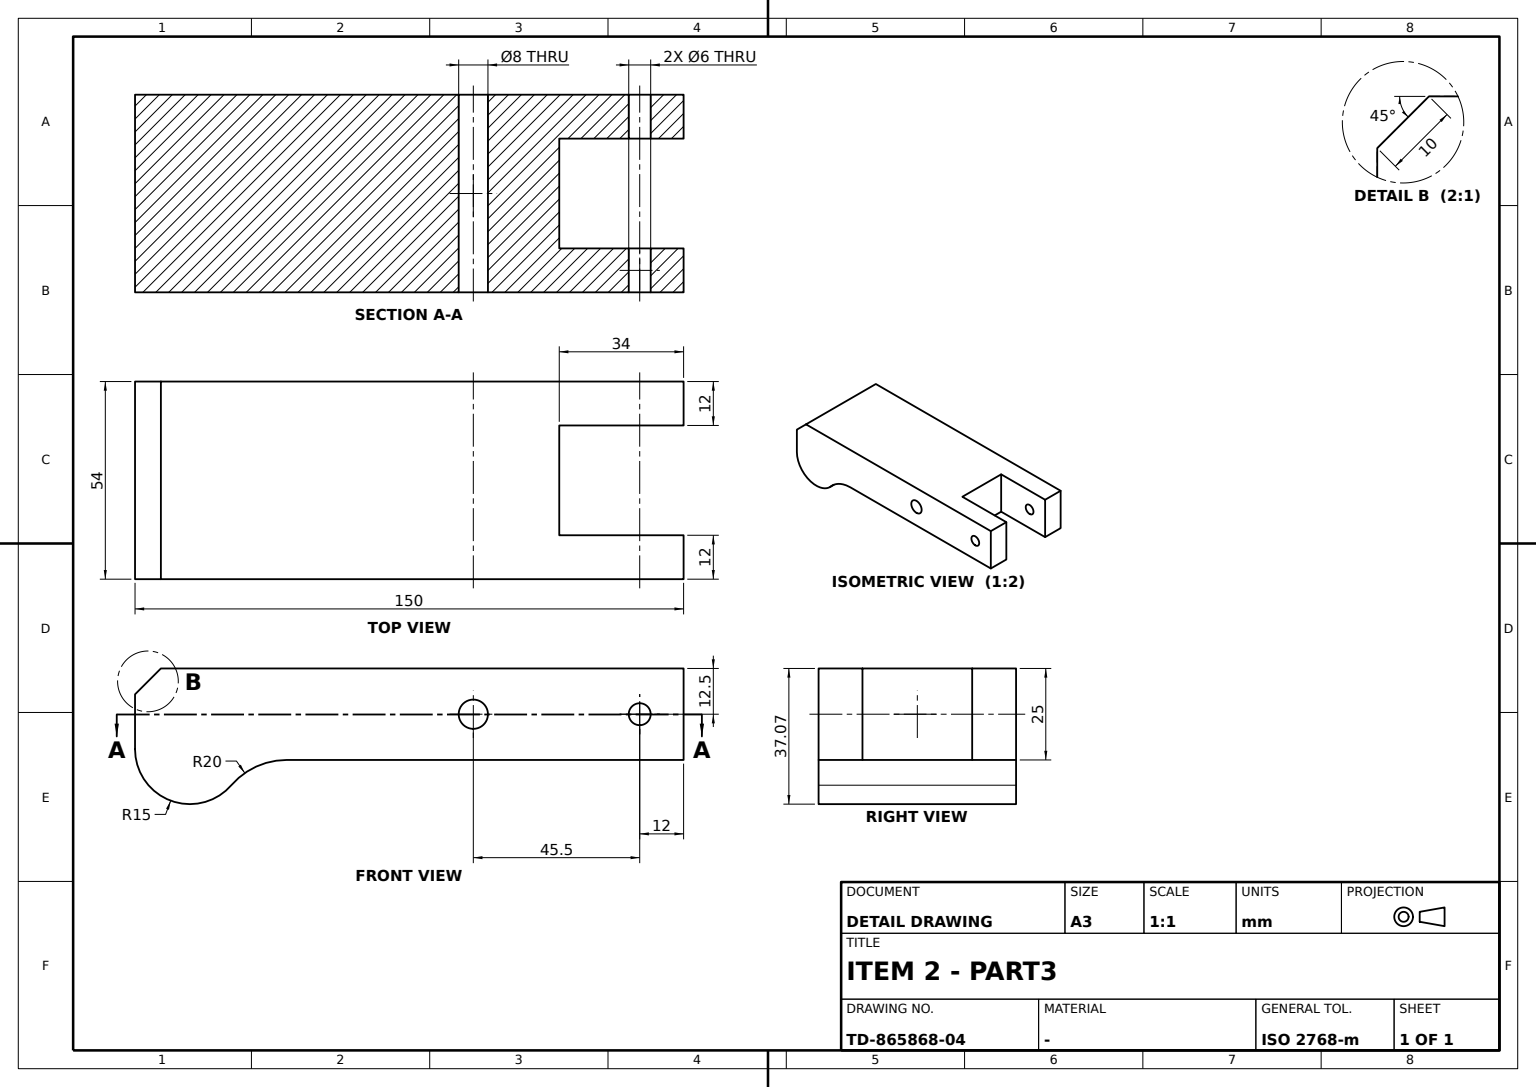
ISO-10303-21;
HEADER;
FILE_DESCRIPTION((''),'2;1');
FILE_NAME('','',(''),(''),'','','');
FILE_SCHEMA(('AUTOMOTIVE_DESIGN'));
ENDSEC;
DATA;
#1=APPLICATION_CONTEXT('');
#2=PRODUCT_CONTEXT('',#1,'mechanical');
#3=PRODUCT('','','',(#2));
#4=PRODUCT_DEFINITION_FORMATION('','',#3);
#5=PRODUCT_DEFINITION_CONTEXT('',#1,'design');
#6=PRODUCT_DEFINITION('','',#4,#5);
#7=PRODUCT_DEFINITION_SHAPE('','',#6);
#8=(LENGTH_UNIT()NAMED_UNIT(*)SI_UNIT(.MILLI.,.METRE.));
#9=(NAMED_UNIT(*)PLANE_ANGLE_UNIT()SI_UNIT($,.RADIAN.));
#10=(NAMED_UNIT(*)SI_UNIT($,.STERADIAN.)SOLID_ANGLE_UNIT());
#11=UNCERTAINTY_MEASURE_WITH_UNIT(LENGTH_MEASURE(0.005),#8,'distance_accuracy_value','');
#12=(GEOMETRIC_REPRESENTATION_CONTEXT(3)GLOBAL_UNCERTAINTY_ASSIGNED_CONTEXT((#11))GLOBAL_UNIT_ASSIGNED_CONTEXT((#8,#9,#10))REPRESENTATION_CONTEXT('',''));
#13=CARTESIAN_POINT('',(27.,77.5,5.571068));
#14=VERTEX_POINT('',#13);
#15=CARTESIAN_POINT('',(27.,77.5,9.571068));
#16=DIRECTION('',(1.,0.,0.));
#17=DIRECTION('',(0.,0.,-1.));
#18=AXIS2_PLACEMENT_3D('',#15,#16,#17);
#19=CIRCLE('',#18,4.);
#20=EDGE_CURVE('',#14,#14,#19,.T.);
#21=ORIENTED_EDGE('',*,*,#20,.T.);
#22=EDGE_LOOP('',(#21));
#23=FACE_BOUND('',#22,.T.);
#24=CARTESIAN_POINT('',(-27.,77.5,5.571068));
#25=VERTEX_POINT('',#24);
#26=CARTESIAN_POINT('',(-27.,77.5,9.571068));
#27=AXIS2_PLACEMENT_3D('',#26,#16,#17);
#28=CIRCLE('',#27,4.);
#29=EDGE_CURVE('',#25,#25,#28,.T.);
#30=ORIENTED_EDGE('',*,*,#29,.F.);
#31=EDGE_LOOP('',(#30));
#32=FACE_BOUND('',#31,.T.);
#33=CARTESIAN_POINT('',(-0.66,77.5,9.571068));
#34=DIRECTION('',(0.,1.,0.));
#35=AXIS2_PLACEMENT_3D('',#33,#16,#34);
#36=CYLINDRICAL_SURFACE('',#35,4.);
#37=ADVANCED_FACE('',(#23,#32),#36,.F.);
#38=CARTESIAN_POINT('',(15.,101.,22.071068));
#39=VERTEX_POINT('',#38);
#40=CARTESIAN_POINT('',(15.,101.,-2.928932));
#41=VERTEX_POINT('',#40);
#42=VECTOR('',#17,1000.);
#43=LINE('',#38,#42);
#44=EDGE_CURVE('',#39,#41,#43,.T.);
#45=ORIENTED_EDGE('',*,*,#44,.T.);
#46=CARTESIAN_POINT('',(-15.,101.,-2.928932));
#47=VERTEX_POINT('',#46);
#48=DIRECTION('',(-1.,0.,0.));
#49=VECTOR('',#48,1000.);
#50=LINE('',#40,#49);
#51=EDGE_CURVE('',#41,#47,#50,.T.);
#52=ORIENTED_EDGE('',*,*,#51,.T.);
#53=CARTESIAN_POINT('',(-15.,101.,22.071068));
#54=VERTEX_POINT('',#53);
#55=LINE('',#53,#42);
#56=EDGE_CURVE('',#54,#47,#55,.T.);
#57=ORIENTED_EDGE('',*,*,#56,.F.);
#58=CARTESIAN_POINT('',(0.,101.,22.071068));
#59=LINE('',#58,#49);
#60=EDGE_CURVE('',#39,#54,#59,.T.);
#61=ORIENTED_EDGE('',*,*,#60,.F.);
#62=EDGE_LOOP('',(#45,#52,#57,#61));
#63=FACE_BOUND('',#62,.T.);
#64=DIRECTION('',(0.,-1.,0.));
#65=AXIS2_PLACEMENT_3D('',#38,#64,#48);
#66=PLANE('',#65);
#67=ADVANCED_FACE('',(#63),#66,.F.);
#68=CARTESIAN_POINT('',(15.,135.,-2.928932));
#69=VERTEX_POINT('',#68);
#70=CARTESIAN_POINT('',(27.,135.,-2.928932));
#71=VERTEX_POINT('',#70);
#72=CARTESIAN_POINT('',(0.,135.,-2.928932));
#73=VECTOR('',#16,1000.);
#74=LINE('',#72,#73);
#75=EDGE_CURVE('',#69,#71,#74,.T.);
#76=ORIENTED_EDGE('',*,*,#75,.T.);
#77=CARTESIAN_POINT('',(27.,26.443602,-2.928932));
#78=VERTEX_POINT('',#77);
#79=CARTESIAN_POINT('',(27.,0.,-2.928932));
#80=VECTOR('',#64,1000.);
#81=LINE('',#79,#80);
#82=EDGE_CURVE('',#71,#78,#81,.T.);
#83=ORIENTED_EDGE('',*,*,#82,.T.);
#84=CARTESIAN_POINT('',(-27.,26.443602,-2.928932));
#85=VERTEX_POINT('',#84);
#86=CARTESIAN_POINT('',(0.,26.443602,-2.928932));
#87=LINE('',#86,#73);
#88=EDGE_CURVE('',#85,#78,#87,.T.);
#89=ORIENTED_EDGE('',*,*,#88,.F.);
#90=CARTESIAN_POINT('',(-27.,135.,-2.928932));
#91=VERTEX_POINT('',#90);
#92=CARTESIAN_POINT('',(-27.,0.,-2.928932));
#93=LINE('',#92,#80);
#94=EDGE_CURVE('',#91,#85,#93,.T.);
#95=ORIENTED_EDGE('',*,*,#94,.F.);
#96=CARTESIAN_POINT('',(-15.,135.,-2.928932));
#97=VERTEX_POINT('',#96);
#98=EDGE_CURVE('',#91,#97,#74,.T.);
#99=ORIENTED_EDGE('',*,*,#98,.T.);
#100=LINE('',#96,#80);
#101=EDGE_CURVE('',#97,#47,#100,.T.);
#102=ORIENTED_EDGE('',*,*,#101,.T.);
#103=ORIENTED_EDGE('',*,*,#51,.F.);
#104=LINE('',#68,#80);
#105=EDGE_CURVE('',#69,#41,#104,.T.);
#106=ORIENTED_EDGE('',*,*,#105,.F.);
#107=EDGE_LOOP('',(#76,#83,#89,#95,#99,#102,#103,#106));
#108=FACE_BOUND('',#107,.T.);
#109=DIRECTION('',(0.,0.,1.));
#110=AXIS2_PLACEMENT_3D('',#72,#109,#64);
#111=PLANE('',#110);
#112=ADVANCED_FACE('',(#108),#111,.F.);
#113=CARTESIAN_POINT('',(27.,-15.,15.));
#114=VERTEX_POINT('',#113);
#115=CARTESIAN_POINT('',(27.,-7.928932,22.071068));
#116=VERTEX_POINT('',#115);
#117=DIRECTION('',(0.,0.707106781,0.707106781));
#118=VECTOR('',#117,1000.);
#119=LINE('',#113,#118);
#120=EDGE_CURVE('',#114,#116,#119,.T.);
#121=ORIENTED_EDGE('',*,*,#120,.T.);
#122=CARTESIAN_POINT('',(-27.,-7.928932,22.071068));
#123=VERTEX_POINT('',#122);
#124=CARTESIAN_POINT('',(0.,-7.928932,22.071068));
#125=LINE('',#124,#73);
#126=EDGE_CURVE('',#123,#116,#125,.T.);
#127=ORIENTED_EDGE('',*,*,#126,.F.);
#128=CARTESIAN_POINT('',(-27.,-15.,15.));
#129=VERTEX_POINT('',#128);
#130=LINE('',#128,#118);
#131=EDGE_CURVE('',#129,#123,#130,.T.);
#132=ORIENTED_EDGE('',*,*,#131,.F.);
#133=CARTESIAN_POINT('',(0.,-15.,15.));
#134=LINE('',#133,#73);
#135=EDGE_CURVE('',#129,#114,#134,.T.);
#136=ORIENTED_EDGE('',*,*,#135,.T.);
#137=EDGE_LOOP('',(#121,#127,#132,#136));
#138=FACE_BOUND('',#137,.T.);
#139=DIRECTION('',(0.,0.707106781,-0.707106781));
#140=AXIS2_PLACEMENT_3D('',#133,#139,#117);
#141=PLANE('',#140);
#142=ADVANCED_FACE('',(#138),#141,.F.);
#143=CARTESIAN_POINT('',(-27.,123.,6.571068));
#144=VERTEX_POINT('',#143);
#145=CARTESIAN_POINT('',(-27.,123.,9.571068));
#146=AXIS2_PLACEMENT_3D('',#145,#16,#17);
#147=CIRCLE('',#146,3.);
#148=EDGE_CURVE('',#144,#144,#147,.T.);
#149=ORIENTED_EDGE('',*,*,#148,.T.);
#150=EDGE_LOOP('',(#149));
#151=FACE_BOUND('',#150,.T.);
#152=CARTESIAN_POINT('',(-27.,135.,22.071068));
#153=VERTEX_POINT('',#152);
#154=CARTESIAN_POINT('',(-27.,0.,22.071068));
#155=VECTOR('',#34,1000.);
#156=LINE('',#154,#155);
#157=EDGE_CURVE('',#123,#153,#156,.T.);
#158=ORIENTED_EDGE('',*,*,#157,.T.);
#159=CARTESIAN_POINT('',(-27.,135.,0.));
#160=LINE('',#159,#42);
#161=EDGE_CURVE('',#153,#91,#160,.T.);
#162=ORIENTED_EDGE('',*,*,#161,.T.);
#163=ORIENTED_EDGE('',*,*,#94,.T.);
#164=CARTESIAN_POINT('',(-27.,11.332972,-9.826685));
#165=VERTEX_POINT('',#164);
#166=CARTESIAN_POINT('',(-27.,26.443602,-22.928932));
#167=AXIS2_PLACEMENT_3D('',#166,#16,#17);
#168=CIRCLE('',#167,20.);
#169=EDGE_CURVE('',#85,#165,#168,.T.);
#170=ORIENTED_EDGE('',*,*,#169,.T.);
#171=CARTESIAN_POINT('',(-27.,-15.,0.));
#172=VERTEX_POINT('',#171);
#173=CARTESIAN_POINT('',(-27.,0.,0.));
#174=AXIS2_PLACEMENT_3D('',#173,#16,#17);
#175=CIRCLE('',#174,15.);
#176=EDGE_CURVE('',#172,#165,#175,.T.);
#177=ORIENTED_EDGE('',*,*,#176,.F.);
#178=VECTOR('',#109,1000.);
#179=LINE('',#171,#178);
#180=EDGE_CURVE('',#172,#129,#179,.T.);
#181=ORIENTED_EDGE('',*,*,#180,.T.);
#182=ORIENTED_EDGE('',*,*,#131,.T.);
#183=EDGE_LOOP('',(#158,#162,#163,#170,#177,#181,#182));
#184=FACE_BOUND('',#183,.T.);
#185=ORIENTED_EDGE('',*,*,#29,.T.);
#186=EDGE_LOOP('',(#185));
#187=FACE_BOUND('',#186,.T.);
#188=AXIS2_PLACEMENT_3D('',#173,#16,#34);
#189=PLANE('',#188);
#190=ADVANCED_FACE('',(#151,#184,#187),#189,.F.);
#191=ORIENTED_EDGE('',*,*,#56,.T.);
#192=ORIENTED_EDGE('',*,*,#101,.F.);
#193=CARTESIAN_POINT('',(-15.,135.,22.071068));
#194=VERTEX_POINT('',#193);
#195=LINE('',#193,#42);
#196=EDGE_CURVE('',#194,#97,#195,.T.);
#197=ORIENTED_EDGE('',*,*,#196,.F.);
#198=CARTESIAN_POINT('',(-15.,-7.928932,22.071068));
#199=LINE('',#198,#155);
#200=EDGE_CURVE('',#54,#194,#199,.T.);
#201=ORIENTED_EDGE('',*,*,#200,.F.);
#202=EDGE_LOOP('',(#191,#192,#197,#201));
#203=FACE_BOUND('',#202,.T.);
#204=CARTESIAN_POINT('',(-15.,123.,12.571068));
#205=VERTEX_POINT('',#204);
#206=CARTESIAN_POINT('',(-15.,123.,9.571068));
#207=AXIS2_PLACEMENT_3D('',#206,#48,#109);
#208=CIRCLE('',#207,3.);
#209=EDGE_CURVE('',#205,#205,#208,.T.);
#210=ORIENTED_EDGE('',*,*,#209,.T.);
#211=EDGE_LOOP('',(#210));
#212=FACE_BOUND('',#211,.T.);
#213=AXIS2_PLACEMENT_3D('',#53,#48,#34);
#214=PLANE('',#213);
#215=ADVANCED_FACE('',(#203,#212),#214,.F.);
#216=ORIENTED_EDGE('',*,*,#209,.F.);
#217=EDGE_LOOP('',(#216));
#218=FACE_BOUND('',#217,.T.);
#219=ORIENTED_EDGE('',*,*,#148,.F.);
#220=EDGE_LOOP('',(#219));
#221=FACE_BOUND('',#220,.T.);
#222=CARTESIAN_POINT('',(-0.66,123.,9.571068));
#223=AXIS2_PLACEMENT_3D('',#222,#16,#34);
#224=CYLINDRICAL_SURFACE('',#223,3.);
#225=ADVANCED_FACE('',(#218,#221),#224,.F.);
#226=CARTESIAN_POINT('',(15.,135.,22.071068));
#227=VERTEX_POINT('',#226);
#228=CARTESIAN_POINT('',(27.,135.,22.071068));
#229=VERTEX_POINT('',#228);
#230=CARTESIAN_POINT('',(0.,135.,22.071068));
#231=LINE('',#230,#73);
#232=EDGE_CURVE('',#227,#229,#231,.T.);
#233=ORIENTED_EDGE('',*,*,#232,.T.);
#234=CARTESIAN_POINT('',(27.,135.,0.));
#235=LINE('',#234,#42);
#236=EDGE_CURVE('',#229,#71,#235,.T.);
#237=ORIENTED_EDGE('',*,*,#236,.T.);
#238=ORIENTED_EDGE('',*,*,#75,.F.);
#239=LINE('',#226,#42);
#240=EDGE_CURVE('',#227,#69,#239,.T.);
#241=ORIENTED_EDGE('',*,*,#240,.F.);
#242=EDGE_LOOP('',(#233,#237,#238,#241));
#243=FACE_BOUND('',#242,.T.);
#244=AXIS2_PLACEMENT_3D('',#230,#64,#17);
#245=PLANE('',#244);
#246=ADVANCED_FACE('',(#243),#245,.F.);
#247=EDGE_CURVE('',#153,#194,#231,.T.);
#248=ORIENTED_EDGE('',*,*,#247,.F.);
#249=ORIENTED_EDGE('',*,*,#157,.F.);
#250=ORIENTED_EDGE('',*,*,#126,.T.);
#251=CARTESIAN_POINT('',(27.,0.,22.071068));
#252=LINE('',#251,#155);
#253=EDGE_CURVE('',#116,#229,#252,.T.);
#254=ORIENTED_EDGE('',*,*,#253,.T.);
#255=ORIENTED_EDGE('',*,*,#232,.F.);
#256=CARTESIAN_POINT('',(15.,-7.928932,22.071068));
#257=LINE('',#256,#80);
#258=EDGE_CURVE('',#227,#39,#257,.T.);
#259=ORIENTED_EDGE('',*,*,#258,.T.);
#260=ORIENTED_EDGE('',*,*,#60,.T.);
#261=ORIENTED_EDGE('',*,*,#200,.T.);
#262=EDGE_LOOP('',(#248,#249,#250,#254,#255,#259,#260,#261));
#263=FACE_BOUND('',#262,.T.);
#264=AXIS2_PLACEMENT_3D('',#124,#17,#34);
#265=PLANE('',#264);
#266=ADVANCED_FACE('',(#263),#265,.F.);
#267=ORIENTED_EDGE('',*,*,#98,.F.);
#268=ORIENTED_EDGE('',*,*,#161,.F.);
#269=ORIENTED_EDGE('',*,*,#247,.T.);
#270=ORIENTED_EDGE('',*,*,#196,.T.);
#271=EDGE_LOOP('',(#267,#268,#269,#270));
#272=FACE_BOUND('',#271,.T.);
#273=ADVANCED_FACE('',(#272),#245,.F.);
#274=CARTESIAN_POINT('',(27.,123.,6.571068));
#275=VERTEX_POINT('',#274);
#276=CARTESIAN_POINT('',(27.,123.,9.571068));
#277=AXIS2_PLACEMENT_3D('',#276,#16,#17);
#278=CIRCLE('',#277,3.);
#279=EDGE_CURVE('',#275,#275,#278,.T.);
#280=ORIENTED_EDGE('',*,*,#279,.F.);
#281=EDGE_LOOP('',(#280));
#282=FACE_BOUND('',#281,.T.);
#283=CARTESIAN_POINT('',(27.,11.332972,-9.826685));
#284=VERTEX_POINT('',#283);
#285=CARTESIAN_POINT('',(27.,26.443602,-22.928932));
#286=AXIS2_PLACEMENT_3D('',#285,#16,#17);
#287=CIRCLE('',#286,20.);
#288=EDGE_CURVE('',#78,#284,#287,.T.);
#289=ORIENTED_EDGE('',*,*,#288,.F.);
#290=ORIENTED_EDGE('',*,*,#82,.F.);
#291=ORIENTED_EDGE('',*,*,#236,.F.);
#292=ORIENTED_EDGE('',*,*,#253,.F.);
#293=ORIENTED_EDGE('',*,*,#120,.F.);
#294=CARTESIAN_POINT('',(27.,-15.,0.));
#295=VERTEX_POINT('',#294);
#296=LINE('',#294,#178);
#297=EDGE_CURVE('',#295,#114,#296,.T.);
#298=ORIENTED_EDGE('',*,*,#297,.F.);
#299=CARTESIAN_POINT('',(27.,0.,0.));
#300=AXIS2_PLACEMENT_3D('',#299,#16,#17);
#301=CIRCLE('',#300,15.);
#302=EDGE_CURVE('',#295,#284,#301,.T.);
#303=ORIENTED_EDGE('',*,*,#302,.T.);
#304=EDGE_LOOP('',(#289,#290,#291,#292,#293,#298,#303));
#305=FACE_BOUND('',#304,.T.);
#306=ORIENTED_EDGE('',*,*,#20,.F.);
#307=EDGE_LOOP('',(#306));
#308=FACE_BOUND('',#307,.T.);
#309=AXIS2_PLACEMENT_3D('',#299,#16,#34);
#310=PLANE('',#309);
#311=ADVANCED_FACE('',(#282,#305,#308),#310,.T.);
#312=ORIENTED_EDGE('',*,*,#169,.F.);
#313=ORIENTED_EDGE('',*,*,#88,.T.);
#314=ORIENTED_EDGE('',*,*,#288,.T.);
#315=CARTESIAN_POINT('',(0.,11.332972,-9.826685));
#316=LINE('',#315,#73);
#317=EDGE_CURVE('',#165,#284,#316,.T.);
#318=ORIENTED_EDGE('',*,*,#317,.F.);
#319=EDGE_LOOP('',(#312,#313,#314,#318));
#320=FACE_BOUND('',#319,.T.);
#321=CARTESIAN_POINT('',(0.,26.443602,-22.928932));
#322=AXIS2_PLACEMENT_3D('',#321,#16,#34);
#323=CYLINDRICAL_SURFACE('',#322,20.);
#324=ADVANCED_FACE('',(#320),#323,.F.);
#325=ORIENTED_EDGE('',*,*,#135,.F.);
#326=ORIENTED_EDGE('',*,*,#180,.F.);
#327=CARTESIAN_POINT('',(0.,-15.,0.));
#328=LINE('',#327,#73);
#329=EDGE_CURVE('',#172,#295,#328,.T.);
#330=ORIENTED_EDGE('',*,*,#329,.T.);
#331=ORIENTED_EDGE('',*,*,#297,.T.);
#332=EDGE_LOOP('',(#325,#326,#330,#331));
#333=FACE_BOUND('',#332,.T.);
#334=AXIS2_PLACEMENT_3D('',#327,#34,#109);
#335=PLANE('',#334);
#336=ADVANCED_FACE('',(#333),#335,.F.);
#337=ORIENTED_EDGE('',*,*,#176,.T.);
#338=ORIENTED_EDGE('',*,*,#317,.T.);
#339=ORIENTED_EDGE('',*,*,#302,.F.);
#340=ORIENTED_EDGE('',*,*,#329,.F.);
#341=EDGE_LOOP('',(#337,#338,#339,#340));
#342=FACE_BOUND('',#341,.T.);
#343=CARTESIAN_POINT('',(0.,0.,0.));
#344=AXIS2_PLACEMENT_3D('',#343,#16,#34);
#345=CYLINDRICAL_SURFACE('',#344,15.);
#346=ADVANCED_FACE('',(#342),#345,.T.);
#347=ORIENTED_EDGE('',*,*,#279,.T.);
#348=EDGE_LOOP('',(#347));
#349=FACE_BOUND('',#348,.T.);
#350=CARTESIAN_POINT('',(15.,123.,6.571068));
#351=VERTEX_POINT('',#350);
#352=CARTESIAN_POINT('',(15.,123.,9.571068));
#353=AXIS2_PLACEMENT_3D('',#352,#16,#17);
#354=CIRCLE('',#353,3.);
#355=EDGE_CURVE('',#351,#351,#354,.T.);
#356=ORIENTED_EDGE('',*,*,#355,.F.);
#357=EDGE_LOOP('',(#356));
#358=FACE_BOUND('',#357,.T.);
#359=ADVANCED_FACE('',(#349,#358),#224,.F.);
#360=ORIENTED_EDGE('',*,*,#240,.T.);
#361=ORIENTED_EDGE('',*,*,#105,.T.);
#362=ORIENTED_EDGE('',*,*,#44,.F.);
#363=ORIENTED_EDGE('',*,*,#258,.F.);
#364=EDGE_LOOP('',(#360,#361,#362,#363));
#365=FACE_BOUND('',#364,.T.);
#366=ORIENTED_EDGE('',*,*,#355,.T.);
#367=EDGE_LOOP('',(#366));
#368=FACE_BOUND('',#367,.T.);
#369=AXIS2_PLACEMENT_3D('',#226,#16,#64);
#370=PLANE('',#369);
#371=ADVANCED_FACE('',(#365,#368),#370,.F.);
#372=CLOSED_SHELL('',(#37,#67,#112,#142,#190,#215,#225,#246,#266,#273,#311,#324,#336,#346,#359,#371));
#373=MANIFOLD_SOLID_BREP('',#372);
#374=ADVANCED_BREP_SHAPE_REPRESENTATION('',(#373),#12);
#375=SHAPE_DEFINITION_REPRESENTATION(#7,#374);
ENDSEC;
END-ISO-10303-21;
